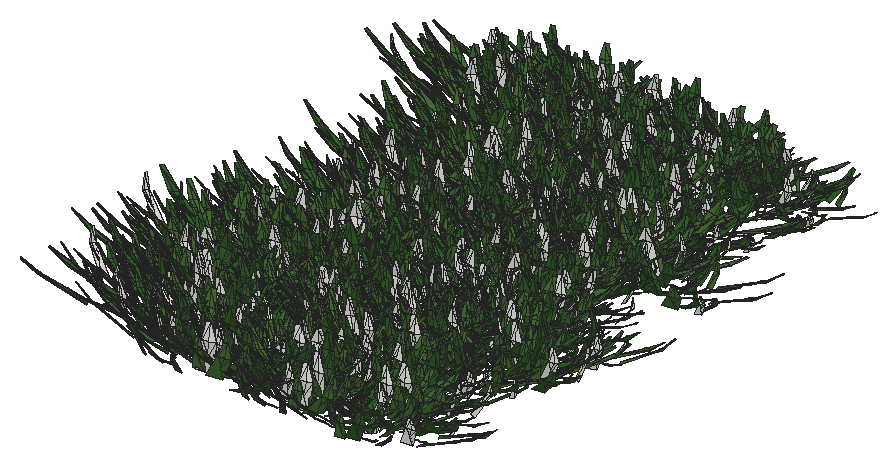
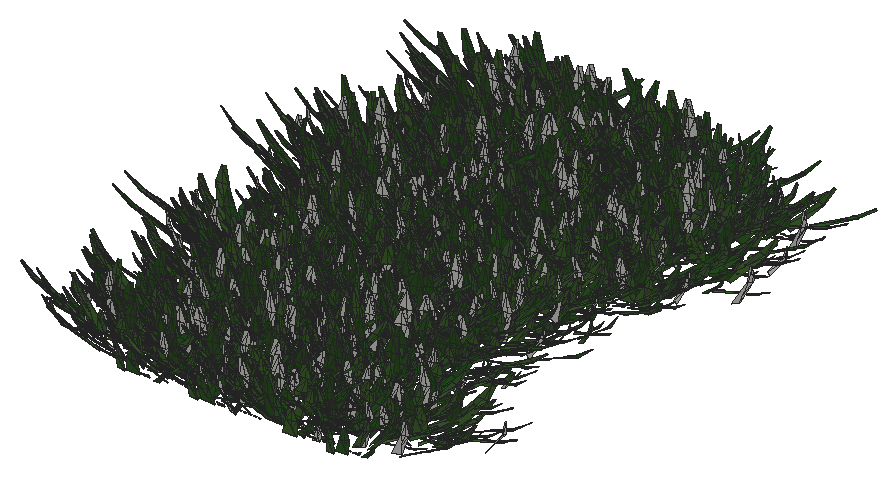
# SketchUp Ruby script. Lengths in inches.
U = 1.inch
M = Sketchup.active_model
def pt(a) = Geom::Point3d.new(a.map { |v| v * U })
def face(e, loops, mat)
  f = e.add_face(loops[0].map { |a| pt(a) })
  loops[1..].each { |l| e.add_face(l.map { |a| pt(a) }).erase! }
  f.material = f.back_material = mat if mat
  f
end
# faces: each face lists its corners as indices into pts; further lists are holes
def faces(e, pts, list, mat = nil) = list.each { |f| face(e, (f[0].is_a?(Array) ? f : [f]).map { |l| l.map { |i| pts[i] } }, mat) }
# xy, xz, yz: faces in a plane at the given z, y or x. An outline is a flat list of corners, or four numbers for a rectangle; further outlines are holes
def ring(l) = l.size == 4 ? [[l[0], l[1]], [l[2], l[1]], [l[2], l[3]], [l[0], l[3]]] : l.each_slice(2).to_a
def flat(e, list, mat, &to3) = list.each { |f| face(e, (f[0].is_a?(Array) ? f : [f]).map { |l| ring(l).map { |u, v| to3.(u, v) } }, mat) }
def xy(e, z, list, mat = nil) = flat(e, list, mat) { |x, y| [x, y, z] }
def xz(e, y, list, mat = nil) = flat(e, list, mat) { |x, z| [x, y, z] }
def yz(e, x, list, mat = nil) = flat(e, list, mat) { |y, z| [x, y, z] }
def lines(e, pts, list) = list.each { |a, b| e.add_line(pt(pts[a]), pt(pts[b])) }
# prism: a flat outline (further loops are holes) pulled along v
def prism(e, loops, v, mat = nil)
  f = face(e, loops, mat); d = Geom::Vector3d.new(v.map { |x| x * U })
  f.pushpull(f.normal.samedirection?(d) ? d.length : -d.length)
end
def box(e, o, s, mat = nil) = prism(e, [[o, [o[0] + s[0], o[1], o[2]], [o[0] + s[0], o[1] + s[1], o[2]], [o[0], o[1] + s[1], o[2]]]], [0, 0, s[2]], mat)
def at(x, y, z, deg = 0) = Geom::Transformation.translation(pt([x, y, z])) * Geom::Transformation.rotation(ORIGIN, Z_AXIS, deg.degrees)
def axes(o, x, y, z) = Geom::Transformation.new([*x, 0, *y, 0, *z, 0, *pt(o).to_a, 1])
def part(name) = M.definitions.add(name)
# library, detail: a bought-in or finely detailed component or shape, given as its bounding box
def library(name, o, s) = part(name).tap { |d| box(d.entities, o, s) }
def detail(e, o, s) = box(e.add_group.entities, o, s)
def put(e, d, t, mat = nil) = e.add_instance(d, t).tap { |i| i.material = mat if mat }
def group(e, t, mat = nil) = e.add_group.tap { |g| g.transformation = t; g.material = mat if mat }.entities
root = M.entities
M.materials.add("Material82").color = [68, 110, 58]
M.materials.add("Material83").color = [48, 90, 38]
M.materials.add("Material84").color = [68, 110, 48]
M.materials.add("Material85").color = [48, 90, 48]
M.materials.add("Material86").color = [58, 110, 58]
M.materials.add("Material87").color = [58, 90, 38]
M.materials.add("Material88").color = [68, 100, 58]
M.materials.add("Material89").color = [48, 100, 38]
c1 = part("grass00")
p = [[-0.6875,0.15,0],[-0.56,0.08,5.52],[-0.04,0.03,2.76],[0.48,-0.02,0],[0.35,-0.02,5.52],[-0.1,-0.14,5.52],
  [-0.12,0.65,8.37],[-0.42,0.65,8.37]]
faces(c1.entities,p,[[0,1,2,3],[3,2,4],[1,5,2],[5,4,2],[1,6,5],[4,5,6],[7,6,1]])
c2 = part("Group16\#1")
put(c2.entities,c1,axes([1.44,-0.61,-0.01],[0.05352,0.12609,0],[-0.10704,0.04543,0.07239],[0.06664,-0.02828,0.11628]),"Material85")
put(c2.entities,c1,axes([0.76,-0.15,-0.01],[0.04676,0.24062,0],[-0.23162,0.04501,0.06642],[0.0652,-0.01267,0.23595]),"Material82")
put(c2.entities,c1,axes([0.79,0.01,-0.01],[-0.00606,0.34651,0],[-0.34381,-0.00602,0.0432],[0.04319,0.00076,0.34386]))
put(c2.entities,c1,axes([1,0.23,-0.01],[-0.07192,0.31144,0],[-0.28722,-0.06632,0.1236],[0.12043,0.02781,0.29478]),"Material84")
put(c2.entities,c1,axes([1.66,0.77,-0.01],[-0.13828,0.29651,0],[-0.21551,-0.1005,0.22471],[0.20365,0.09498,0.23779]),"Material89")
put(c2.entities,c1,axes([0.6875,0.52,-0.01],[-0.18126,0.24051,0],[-0.22746,-0.17142,0.09788],[0.07817,0.05891,0.28481]),"Material84")
put(c2.entities,c1,axes([0.68,0.78,-0.01],[-0.215,0.18688,0],[-0.12385,-0.14248,0.21334],[0.13995,0.16101,0.18878]),"Material82")
put(c2.entities,c1,axes([0.56,1,-0.01],[-0.13756,0.07624,0],[-0.06159,-0.11112,0.0927],[0.04494,0.08108,0.12705]),"Material84")
put(c2.entities,c1,axes([0.2,0.64,-0.01],[-0.23729,0.07254,0],[-0.05711,-0.18681,0.153],[0.04473,0.14632,0.19535]),"Material89")
put(c2.entities,c1,axes([0.0625,0.72,-0.01],[-0.28874,0.02525,0],[-0.02179,-0.24916,0.14647],[0.01276,0.14591,0.25012]),"Material82")
put(c2.entities,c1,axes([-0.08,0.62,-0.01],[-0.34089,-0.04187,0],[0.03255,-0.26504,0.216],[-0.02633,0.21439,0.26703]),"Material89")
put(c2.entities,c1,axes([-0.34,0.98,-0.01],[-0.14314,-0.0493,0],[0.04397,-0.12769,0.06843],[-0.02228,0.0647,0.13505]),"Material89")
put(c2.entities,c1,axes([-0.87,1.45,-0.01],[-0.23488,-0.14114,0],[0.13761,-0.22901,0.06087],[-0.03135,0.05217,0.26717]))
put(c2.entities,c1,axes([-0.72,0.77,-0.01],[-0.14208,-0.13251,0],[0.07209,-0.0773,0.16301],[-0.11118,0.11922,0.1057]),"Material89")
put(c2.entities,c1,axes([-0.62,0.43,-0.01],[-0.14845,-0.21203,0],[0.18654,-0.13061,0.12304],[-0.10079,0.07057,0.22772]),"Material82")
put(c2.entities,c1,axes([-0.68,0.29,-0.01],[-0.13639,-0.32136,0],[0.31723,-0.13464,0.05579],[-0.05136,0.0218,0.34462]),"Material83")
put(c2.entities,c1,axes([-0.64,0.125,-0.01],[-0.0458,-0.23569,0],[0.22124,-0.043,0.08276],[-0.08124,0.01579,0.22538]),"Material86")
put(c2.entities,c1,axes([-1.6,-0.03,-0.01],[0.00576,-0.32897,0],[0.27526,0.00482,0.18018],[-0.18015,-0.00315,0.2753]),"Material84")
put(c2.entities,c1,axes([-1.36,-0.31,-0.01],[0.05718,-0.24765,0],[0.18172,0.04196,0.17267],[-0.16825,-0.03885,0.1865]),"Material89")
put(c2.entities,c1,axes([-1.54,-0.72,-0.01],[0.06537,-0.14017,0],[0.13555,0.06321,0.03939],[-0.0357,-0.01665,0.14956]))
put(c2.entities,c1,axes([-1.19,-0.9,-0.01],[0.09597,-0.12735,0],[0.11214,0.08451,0.07557],[-0.06035,-0.04548,0.14042]),"Material88")
put(c2.entities,c1,axes([-0.47,-0.54,-0.01],[0.11588,-0.10072,0],[0.0618,0.0711,0.12124],[-0.07953,-0.0915,0.0942]))
put(c2.entities,c1,axes([-0.47,-0.84,-0.01],[0.11927,-0.0661,0],[0.06603,0.11913,0.00646],[-0.00313,-0.00565,0.13621]),"Material84")
put(c2.entities,c1,axes([-0.38,-1.24,-0.01],[0.28037,-0.08571,0],[0.0618,0.20215,0.20315],[-0.05939,-0.19428,0.21139]),"Material88")
put(c2.entities,c1,axes([-0.06,-0.66,-0.01],[0.22719,-0.01987,0],[0.01247,0.14255,0.17758],[-0.01547,-0.17691,0.1431]),"Material87")
put(c2.entities,c1,axes([0.11,-0.89,-0.01],[0.14882,0.01828,0],[-0.01058,0.08611,0.12229],[0.01491,-0.12138,0.08676]),"Material85")
put(c2.entities,c1,axes([0.25,-0.72,-0.01],[0.20481,0.07053,0],[-0.06206,0.18022,0.10291],[0.03351,-0.0973,0.1906]),"Material85")
put(c2.entities,c1,axes([0.85,-1.42,-0.01],[0.16481,0.09904,0],[-0.09472,0.15762,0.05616],[0.02893,-0.04814,0.18389]),"Material84")
put(c2.entities,c1,axes([1.01,-1.09,-0.01],[0.21858,0.20385,0],[-0.17495,0.1876,0.15339],[0.10462,-0.11218,0.25652]),"Material89")
put(c2.entities,c1,axes([1.01,-0.71,-0.01],[0.08733,0.12473,0],[-0.06445,0.04512,0.13037],[0.1068,-0.07477,0.07867]),"Material85")
c3 = part("Group15\#1")
put(c3.entities,c2,at(0,0,0))
c4 = part("3darcstudiotree_grass00\#1")
put(c4.entities,c3,at(0,0,0))
put(root,c4,axes([1732.73,956.72,-29.74],[2.78328,1.41625,0],[-3.60575,1.10211,-0.03267],[-0.14651,0.04478,1.93988]))
put(root,c4,axes([1732.9,991.06,-29.74],[1.42302,1.52353,0],[-4.19442,0.60932,-0.04046],[-0.17686,0.02569,1.56076]))
put(root,c4,axes([1733,952.4375,-29.74],[0.02685,1.39613,0],[-4.67009,0.01397,-0.03677],[-0.14547,0.00044,1.38481]))
put(root,c4,axes([1734.73,944.23,-29.74],[-3.90096,-0.14279,0],[0.42836,-1.82008,-0.06502],[0.0247,-0.10495,1.42798]))
put(root,c4,axes([1733.78,961.63,-29.74],[-0.58657,1.2788,0],[-3.43074,-0.24475,-0.01415],[-0.07642,-0.00545,1.43376]))
put(root,c4,axes([1734.81,950.95,-29.74],[1.37504,-1.64012,0],[4.21946,0.55019,-0.04027],[0.19656,0.02563,1.71232]))
put(root,c4,axes([1734.89,992.02,-29.74],[3.4755,-0.56156,0],[1.30477,1.25594,-0.00746],[0.01674,0.01612,1.52751]))
put(root,c4,axes([1734.32,945.99,-29.74],[2.831,1.13552,0],[-3.26481,1.26594,-0.00938],[-0.03813,0.01479,1.95578]))
put(root,c4,axes([1737,963.81,-29.74],[-0.94888,-1.39552,0],[4.53946,-0.48005,-0.04199],[0.20499,-0.02168,1.7807]))
put(root,c4,axes([1737.37,970.1875,-29.74],[-2.56412,-1.04956,0],[2.92241,-1.11041,-0.03217],[0.12075,-0.04588,1.58546]))
put(root,c4,axes([1737.06,950.78,-29.74],[-4.23608,0.30685,0],[-0.85226,-1.82987,-0.05609],[-0.05564,-0.11947,1.94158]))
put(root,c4,axes([1737.32,960.52,-29.74],[-3.83901,-0.76558,0],[1.48905,-1.16132,-0.0255],[0.09039,-0.0705,1.94297]))
put(root,c4,axes([1737,996.64,-29.74],[-3.22115,0.33319,0],[-1.15137,-1.73117,-0.03948],[-0.04657,-0.07003,1.58152]))
put(root,c4,axes([1736.98,988.74,-29.74],[-3.56945,0.98002,0],[-2.54129,-1.43957,-0.02528],[-0.0766,-0.04339,1.76765]))
put(root,c4,axes([1736.73,947.1,-29.74],[0.13943,1.51336,0],[-3.52829,0.05056,-0.04285],[-0.2957,0.00424,1.82733]))
put(root,c4,axes([1736.92,986.46,-29.74],[3.38923,-0.39007,0],[1.26949,1.71555,-0.04654],[0.05157,0.06969,1.34343]))
put(root,c4,axes([1736.65,994.52,-29.74],[3.63174,0.64343,0],[-1.49454,1.312,-0.04301],[-0.1083,0.09507,1.6797]))
put(root,c4,axes([1737.22,961.37,-29.74],[3.52935,-0.50726,0],[1.49485,1.61761,-0.06136],[0.11602,0.12555,1.80687]))
put(root,c4,axes([1738.61,948.92,-29.74],[-0.52019,-1.47295,0],[3.61124,-0.19836,-0.01078],[0.07028,-0.00386,1.79898]))
put(root,c4,axes([1738.97,972.49,-29.74],[-1.338,-1.30891,0],[3.60545,-0.57321,-0.00075],[0.00363,-0.00058,1.52674]))
put(root,c4,axes([1737.54,953.74,-29.74],[3.75686,0.07381,0],[-0.21994,1.74119,-0.00527],[-0.00126,0.00998,1.59512]))
put(root,c4,axes([1739.66,992.26,-29.74],[-1.97999,-1.67359,0],[3.87039,-0.71217,-0.01753],[0.07436,-0.01368,1.49864]))
put(root,c4,axes([1738.46,980.1,-29.74],[3.4977,-1.17788,0],[2.34178,1.08154,-0.01134],[0.04108,0.01897,1.5074]))
put(root,c4,axes([1739.2,945.17,-29.74],[-4.29885,0.51765,0],[-1.3445,-1.73657,-0.03433],[-0.03931,-0.05078,1.35329]))
put(root,c4,axes([1738.99,974.28,-29.74],[-3.01219,1.1686,0],[-2.47695,-0.99299,-0.0233],[-0.1132,-0.04538,1.83382]))
put(root,c4,axes([1738.73,977.27,-29.74],[-0.71352,1.56405,0],[-4.14814,-0.29432,-0.02584],[-0.10481,-0.00744,1.30174]))
put(root,c4,axes([1739.89,983.25,-29.74],[1.98892,-1.13086,0],[3.89758,1.06614,-0.02169],[0.07891,0.02158,1.57389]))
put(root,c4,axes([1739.04,955.29,-29.74],[-0.64515,1.28427,0],[-4.09885,-0.32024,-0.03573],[-0.18751,-0.01465,1.67549]))
put(root,c4,axes([1740.4375,941.89,-29.74],[-3.41936,-0.32293,0],[0.80872,-1.33182,-0.00326],[0.00565,-0.00931,1.93944]))
put(root,c4,axes([1738.94,957.94,-29.74],[2.80686,0.98493,0],[-2.35719,1.04478,-0.00943],[-0.03285,0.01456,1.39243]))
put(root,c4,axes([1739.68,965.74,-29.74],[-0.90085,1.67926,0],[-4.44806,-0.37112,-0.05558],[-0.25392,-0.02119,1.59125]))
put(root,c4,axes([1740.39,989.9,-29.74],[1.68218,-1.47179,0],[3.03421,0.53937,-0.02223],[0.13236,0.02353,1.62899]))
put(root,c4,axes([1740.48,980.9,-29.74],[3.50844,-0.55754,0],[1.25662,1.22985,-0.02314],[0.04614,0.04516,1.34449]))
put(root,c4,axes([1739.95,968.23,-29.74],[1.7612,1.59038,0],[-3.40002,0.5856,-0.01938],[-0.1015,0.01748,1.58937]))
put(root,c4,axes([1742.14,960.2,-29.74],[-1.60359,-1.29455,0],[3.30864,-0.63743,-0.0349],[0.20941,-0.04034,1.84302]))
put(root,c4,axes([1742.72,973.52,-29.74],[-3.86108,-0.00922,0],[0.0279,-1.817,-0.0591],[0.00158,-0.1028,1.52309]))
put(root,c4,axes([1742.93,969.26,-29.74],[-4.30049,-0.14117,0],[0.33609,-1.59238,-0.036],[0.01919,-0.09092,1.9513]))
put(root,c4,axes([1742.7,985.21,-29.74],[1.67099,-1.73753,0],[3.10475,0.46439,-0.00605],[0.0444,0.00664,1.95327]))
put(root,c4,axes([1742.79,997.1,-29.74],[1.32812,-1.21732,0],[3.65511,0.62022,-0.02985],[0.14197,0.02409,1.54439]))
put(root,c4,axes([1742.5,980.74,-29.74],[0.83797,-1.39271,0],[3.20742,0.30015,-0.04624],[0.35526,0.03324,1.95114]))
put(root,c4,axes([1742.49,990.49,-29.74],[-2.03219,1.40442,0],[-2.95743,-0.66557,-0.04437],[-0.22116,-0.04977,1.46464]))
put(root,c4,axes([1742.14,948.75,-29.74],[-0.97814,1.51943,0],[-3.80237,-0.3807,-0.01715],[-0.08253,-0.00826,1.46021]))
put(root,c4,axes([1743.71,974.73,-29.74],[-0.67683,-1.69031,0],[4.16932,-0.25965,-0.01303],[0.08012,-0.00499,1.96953]))
put(root,c4,axes([1743.39,940.56,-29.74],[1.22394,-1.54587,0],[4.34445,0.53497,-0.04262],[0.21661,0.02667,1.81655]))
put(root,c4,axes([1743.99,963.42,-29.74],[-4.29208,0.36507,0],[-0.8528,-1.5594,-0.00845],[-0.00798,-0.0146,1.35873]))
put(root,c4,axes([1743.45,953.15,-29.74],[-2.45653,1.59128,0],[-3.13753,-0.75331,-0.03488],[-0.14833,-0.03561,1.37068]))
put(root,c4,axes([1743,958.01,-29.74],[3.38301,-0.17676,0],[0.47183,1.40447,-0.04905],[0.03546,0.10554,1.48186]))
put(root,c4,axes([1743.66,966.33,-29.74],[-2.91157,1.30067,0],[-2.86972,-0.9991,-0.01581],[-0.05499,-0.01914,1.33135]))
put(root,c4,axes([1743.625,945.11,-29.74],[3.20776,-0.47754,0],[1.28857,1.34619,-0.04981],[0.10847,0.11332,1.68613]))
put(root,c4,axes([1744.86,945.81,-29.74],[-0.83396,-1.47678,0],[3.24144,-0.28469,-0.00779],[0.04244,-0.00373,1.38852]))
put(root,c4,axes([1744.88,971.18,-29.74],[-2.06199,-1.44492,0],[3.43124,-0.76156,-0.05229],[0.2544,-0.05646,1.64764]))
put(root,c4,axes([1744.98,955.42,-29.74],[0.41064,-1.32496,0],[4.30887,0.2077,-0.02785],[0.12721,0.00613,1.49696]))
put(root,c4,axes([1744.07,962.01,-29.74],[-2.19345,1.65823,0],[-4.03021,-0.82913,-0.04188],[-0.20563,-0.0423,1.88687]))
put(root,c4,axes([1743.46,983.93,-29.74],[2.88531,0.9286,0],[-2.55752,1.23593,-0.03119],[-0.12387,0.05986,1.90467]))
put(root,c4,axes([1744.59,994.86,-29.74],[-1.83042,1.58988,0],[-3.0568,-0.54735,-0.0444],[-0.26156,-0.04683,1.62807]))
put(root,c4,axes([1744.93,976.625,-29.74],[-2.26778,1.36387,0],[-3.7802,-0.97758,-0.05216],[-0.16857,-0.04359,1.30947]))
put(root,c4,axes([1744.93,978.76,-29.74],[-1.84352,1.61201,0],[-4.26993,-0.75947,-0.03185],[-0.15055,-0.02678,1.82087]))
put(root,c4,axes([1745.02,951.04,-29.74],[2.07706,1.01263,0],[-2.63538,0.84072,-0.02717],[-0.1514,0.0483,1.82093]))
put(root,c4,axes([1745.12,942.21,-29.74],[3.46015,0.38109,0],[-0.88814,1.25417,-0.03829],[-0.05842,0.0825,1.40372]))
put(root,c4,axes([1745.64,988.56,-29.74],[3.97524,-0.29729,0],[0.87691,1.8237,-0.05959],[0.04913,0.10217,1.56123]))
put(root,c4,axes([1745.76,991.9375,-29.74],[0.81482,1.77329,0],[-4.44159,0.31742,-0.02342],[-0.11628,0.00831,1.70718]))
put(root,c4,axes([1747.86,941.86,-29.74],[-3.61082,-0.39433,0],[1.20081,-1.71014,-0.02644],[0.03989,-0.05681,1.9068]))
put(root,c4,axes([1748.57,981.76,-29.74],[-3.88555,-0.79581,0],[2.02489,-1.53765,-0.03725],[0.08107,-0.06156,1.55507]))
put(root,c4,axes([1747.78,994.47,-29.74],[-2.70631,1.45447,0],[-3.636,-1.05223,-0.06171],[-0.25363,-0.0734,1.72322]))
put(root,c4,axes([1747.52,987.51,-29.74],[1.70731,1.1244,0],[-2.88773,0.68196,-0.04808],[-0.30467,0.07195,1.86326]))
put(root,c4,axes([1747.49,970.15,-29.74],[4.38861,-0.21228,0],[0.43057,1.38444,-0.03723],[0.02239,0.072,1.30959]))
put(root,c4,axes([1748.84,990.03,-29.74],[0.3333,-1.68825,0],[3.84573,0.11808,-0.01871],[0.11577,0.00355,1.79426]))
put(root,c4,axes([1749.36,973.2,-29.74],[-2.17802,-1.23467,0],[3.55396,-0.97507,-0.03629],[0.13271,-0.03641,1.44541]))
put(root,c4,axes([1749.45,968.3,-29.74],[-2.33047,-0.97071,0],[3.43186,-1.28143,-0.06171],[0.20646,-0.07709,1.63202]))
put(root,c4,axes([1749.65,946.09,-29.74],[0.8669,-1.63737,0],[4.38165,0.36081,-0.01659],[0.07514,0.00619,1.55232]))
put(root,c4,axes([1750.2,984.53,-29.74],[-4.08688,-0.61044,0],[1.62889,-1.6961,-0.00084],[0.00115,-0.0012,1.34285]))
put(root,c4,axes([1749.41,979.54,-29.74],[-2.729,0.78907,0],[-2.0311,-1.09252,-0.03589],[-0.15909,-0.08558,1.93035]))
put(root,c4,axes([1748.87,977.77,-29.74],[3.45505,-0.2676,0],[0.73895,1.48387,-0.00241],[0.00289,0.0058,1.79003]))
put(root,c4,axes([1749.36,975.52,-29.74],[-1.50877,1.48911,0],[-3.61563,-0.56976,-0.0529],[-0.26655,-0.042,1.58349]))
put(root,c4,axes([1748.85,956.99,-29.74],[1.39252,1.41751,0],[-3.18673,0.48689,-0.02409],[-0.14094,0.02153,1.60735]))
put(root,c4,axes([1748.74,944.65,-29.74],[4.57837,0.42186,0],[-0.79113,1.33536,-0.04207],[-0.04884,0.08244,1.32997]))
put(root,c4,axes([1749.98,952.64,-29.74],[-2.78854,1.36928,0],[-2.88748,-0.91457,-0.04358],[-0.20411,-0.06465,1.66757]))
put(root,c4,axes([1749.28,966.02,-29.74],[3.59081,0.56064,0],[-1.39714,1.39174,-0.03237],[-0.06842,0.06816,1.63378]))
put(root,c4,axes([1750.4,996.53,-29.74],[-3.54904,1.16368,0],[-2.54993,-1.20953,-0.00935],[-0.03236,-0.01535,1.61847]))
put(root,c4,axes([1750.21,963.43,-29.74],[3.39127,-1.14999,0],[2.14538,0.98397,-0.0226],[0.09906,0.04544,1.65792]))
put(root,c4,axes([1751.34,986.53,-29.74],[-4.21718,-0.04667,0],[0.09647,-1.35575,-0.03959],[0.00846,-0.11883,1.96257]))
put(root,c4,axes([1749.8125,962,-29.74],[4.10063,0.83805,0],[-2.12312,1.61572,-0.0509],[-0.10915,0.08307,1.61215]))
put(root,c4,axes([1750.5,960.24,-29.74],[3.6923,-0.26906,0],[0.83055,1.77269,-0.01263],[0.0116,0.02476,1.73191]))
put(root,c4,axes([1751.18,951.2,-29.74],[2.76982,-1.52047,0],[2.85461,0.80878,-0.0087],[0.04308,0.01221,1.60603]))
put(root,c4,axes([1751.42,955.36,-29.74],[3.07151,-0.57195,0],[1.60637,1.34169,-0.03456],[0.08725,0.07287,1.66747]))
put(root,c4,axes([1751.51,991.79,-29.74],[-0.75802,1.26839,0],[-3.28645,-0.30547,-0.04738],[-0.26314,-0.02446,1.4441]))
put(root,c4,axes([1750.82,949.48,-29.74],[2.67266,1.37649,0],[-3.28703,0.99263,-0.02004],[-0.06999,0.02114,1.3651]))
put(root,c4,axes([1753.08,996.91,-29.74],[-3.58911,0.17625,0],[-0.41421,-1.31187,-0.03309],[-0.02615,-0.08283,1.60704]))
put(root,c4,axes([1753.51,977.36,-29.74],[-3.53984,-0.54558,0],[1.35048,-1.36277,-0.02269],[0.0488,-0.04924,1.64292]))
put(root,c4,axes([1753.3,950.69,-29.74],[-4.11453,0.51388,0],[-1.13165,-1.40923,-0.01419],[-0.02668,-0.03323,1.75006]))
put(root,c4,axes([1753.125,940.28,-29.74],[2.17079,-1.3067,0],[3.53732,0.91396,-0.04807],[0.21538,0.05565,1.69791]))
put(root,c4,axes([1753.29,964.18,-29.74],[2.51974,-1.17528,0],[3.05999,1.02034,-0.03628],[0.13748,0.04584,1.49031]))
put(root,c4,axes([1754.1,985.46,-29.74],[-1.7024,-1.44396,0],[3.0538,-0.55996,-0.04244],[0.29035,-0.05324,1.90455]))
put(root,c4,axes([1754.11,942.14,-29.74],[1.63405,-1.64828,0],[3.24927,0.50099,-0.00888],[0.05923,0.00913,1.87213]))
put(root,c4,axes([1753.18,943.67,-29.74],[-1.01765,1.47435,0],[-4.56253,-0.4898,-0.0223],[-0.09653,-0.01036,1.58974]))
put(root,c4,axes([1754.8,992.84,-29.74],[-0.95803,-1.53129,0],[3.44538,-0.33525,-0.01268],[0.07432,-0.00723,1.60602]))
put(root,c4,axes([1755.26,965.75,-29.74],[-1.89774,-1.54823,0],[3.70179,-0.70571,-0.04214],[0.19197,-0.0366,1.55921]))
put(root,c4,axes([1754.53,987.47,-29.74],[-2.99752,0.92431,0],[-2.30263,-1.1614,-0.02144],[-0.09164,-0.04622,1.94421]))
put(root,c4,axes([1753.95,972.62,-29.74],[-0.63419,1.43243,0],[-3.71512,-0.25582,-0.03794],[-0.18856,-0.01298,1.42617]))
put(root,c4,axes([1754.52,948.26,-29.74],[-1.88196,1.3957,0],[-3.10758,-0.65171,-0.04799],[-0.32006,-0.06712,1.99284]))
put(root,c4,axes([1755.56,958.05,-29.74],[-1.98727,-1.58329,0],[3.14557,-0.61406,-0.01272],[0.05955,-0.01163,1.37453]))
put(root,c4,axes([1755.32,994.26,-29.74],[0.20206,-1.72347,0],[4.27325,0.07792,-0.04434],[0.21389,0.0039,1.54852]))
put(root,c4,axes([1756.19,959.95,-29.74],[-2.8282,-0.92386,0],[2.41261,-1.14869,-0.01497],[0.06145,-0.02926,1.82381]))
put(root,c4,axes([1754.75,945.9,-29.74],[-1.66334,1.46333,0],[-4.128,-0.72978,-0.00369],[-0.01567,-0.00277,1.57624]))
put(root,c4,axes([1755.49,955.7,-29.74],[-3.33624,1.28886,0],[-2.34327,-0.94338,-0.00183],[-0.00717,-0.00289,1.40539]))
put(root,c4,axes([1755.31,979.55,-29.74],[-2.28466,1.61729,0],[-3.8326,-0.84205,-0.0557],[-0.22938,-0.0504,1.55009]))
put(root,c4,axes([1756.59,983.32,-29.74],[-3.20918,-1.37059,0],[3.45166,-1.25697,-0.04946],[0.15315,-0.05577,1.48426]))
put(root,c4,axes([1756.4,969.96,-29.74],[-4.01536,-0.24387,0],[0.54359,-1.39202,-0.03709],[0.03558,-0.0911,1.68681]))
put(root,c4,axes([1756.06,968.24,-29.74],[-3.12054,0.56833,0],[-1.82234,-1.55622,-0.05064],[-0.09583,-0.08183,1.47033]))
put(root,c4,axes([1756.8,953.34,-29.74],[0.84647,-1.73268,0],[3.98325,0.30265,-0.00212],[0.01137,0.00086,1.6588]))
put(root,c4,axes([1756.21,990.19,-29.74],[3.17331,-0.50017,0],[1.66687,1.64477,-0.02256],[0.03879,0.03827,1.55958]))
put(root,c4,axes([1756.71,980.79,-29.74],[1.96831,-1.06776,0],[3.09361,0.88694,-0.02782],[0.14847,0.04257,1.89124]))
put(root,c4,axes([1756.17,962.45,-29.74],[2.38559,0.94842,0],[-2.99836,1.17298,-0.03885],[-0.13848,0.05417,1.58937]))
put(root,c4,axes([1756.72,975.67,-29.74],[3.11027,0.45791,0],[-1.48719,1.57105,-0.03179],[-0.06172,0.0652,1.76952]))
put(root,c4,axes([1758.63,970.99,-29.74],[-1.60231,-1.37282,0],[3.29691,-0.59848,-0.04546],[0.27162,-0.04931,1.78943]))
put(root,c4,axes([1758.99,973.1,-29.74],[0.96155,-1.39333,0],[3.31195,0.35548,-0.01758],[0.11319,0.01215,1.71636]))
put(root,c4,axes([1759.36,951.07,-29.74],[-3.63945,-0.58666,0],[1.30533,-1.25945,-0.04864],[0.1019,-0.09832,1.4319]))
put(root,c4,axes([1759.48,980.76,-29.74],[-1.71956,-1.37213,0],[4.12265,-0.80354,-0.04891],[0.23955,-0.04669,1.88309]))
put(root,c4,axes([1759.72,994.17,-29.74],[-3.8816,-0.56323,0],[1.5517,-1.6632,-0.01333],[0.02356,-0.02525,1.7245]))
put(root,c4,axes([1759.05,996.82,-29.74],[-3.46015,1.06405,0],[-2.06953,-1.04669,-0.02241],[-0.08068,-0.04081,1.47722]))
put(root,c4,axes([1759.3,948.7,-29.74],[-0.53843,-1.61653,0],[3.48383,-0.18047,-0.04534],[0.27707,-0.01435,1.62314]))
put(root,c4,axes([1759.68,961.84,-29.74],[0.02414,-1.32822,0],[3.48081,0.00984,-0.01704],[0.11733,0.00033,1.79616]))
put(root,c4,axes([1758.5,991.89,-29.74],[-1.06746,1.42925,0],[-3.87706,-0.45036,-0.01201],[-0.05554,-0.00645,1.46096]))
put(root,c4,axes([1760.08,967.68,-29.74],[-1.25473,-1.49042,0],[3.70912,-0.48565,-0.03393],[0.14523,-0.01902,1.3212]))
put(root,c4,axes([1758.98,940.29,-29.74],[4.07054,-0.47424,0],[1.26442,1.68794,-0.05518],[0.08285,0.1106,1.77288]))
put(root,c4,axes([1760.56,944.52,-29.74],[0.9992,-1.70874,0],[3.78612,0.34433,-0.00305],[0.01806,0.00164,1.76865]))
put(root,c4,axes([1759.75,964.62,-29.74],[-2.38248,1.06709,0],[-3.21771,-1.11734,-0.02335],[-0.09118,-0.03166,1.67208]))
put(root,c4,axes([1759.07,983.89,-29.74],[0.13535,1.36053,0],[-4.14262,0.0641,-0.00595],[-0.03791,0.00059,1.98232]))
put(root,c4,axes([1760.18,985.67,-29.74],[-3.44248,1.19972,0],[-2.84327,-1.26888,-0.04086],[-0.12277,-0.05479,1.46035]))
put(root,c4,axes([1760.42,965.7,-29.74],[2.50615,-1.32245,0],[2.94011,0.86656,-0.03861],[0.1979,0.05833,1.76068]))
put(root,c4,axes([1761.18,945.85,-29.74],[0.83554,-1.66698,0],[4.46376,0.34798,-0.04547],[0.22573,0.0176,1.72572]))
put(root,c4,axes([1760.97,990.65,-29.74],[-3.77371,1.09403,0],[-2.05317,-1.10148,-0.00523],[-0.01755,-0.00942,1.47184]))
put(root,c4,axes([1761,975.46,-29.74],[-3.53362,0.69285,0],[-1.78137,-1.413,-0.01143],[-0.02296,-0.01821,1.35283]))
put(root,c4,axes([1760.12,955.1,-29.74],[3.52761,0.55067,0],[-1.26989,1.26523,-0.04887],[-0.1287,0.12823,1.85053]))
put(root,c4,axes([1762,957.66,-29.74],[-4.29343,-0.7683,0],[1.85419,-1.61153,-0.00153],[0.00342,-0.00297,1.82565]))
put(root,c4,axes([1761.73,942.29,-29.74],[-4.08016,-0.15242,0],[0.34321,-1.42893,-0.02721],[0.0124,-0.05162,1.31849]))
put(root,c4,axes([1760.68,978.6,-29.74],[1.28441,1.48375,0],[-3.48852,0.46968,-0.04031],[-0.24472,0.03295,1.77227]))
put(root,c4,axes([1761.7,988.62,-29.74],[-3.58514,0.47051,0],[-1.41535,-1.67729,-0.02244],[-0.03437,-0.04073,1.62972]))
put(root,c4,axes([1762.03,960.4375,-29.74],[0.26653,-1.73376,0],[4.03869,0.09656,-0.02606],[0.1443,0.00345,1.68211]))
put(root,c4,axes([1761.76,953.66,-29.74],[-2.42435,1.35441,0],[-3.23148,-0.89962,-0.04566],[-0.20763,-0.0578,1.65042]))
put(root,c4,axes([1762.52,977.57,-29.74],[3.81611,-0.29546,0],[0.81359,1.63432,-0.02697],[0.02626,0.05275,1.59996]))
put(root,c4,axes([1764.79,962.01,-29.74],[-4.03021,-0.53258,0],[1.1352,-1.33605,-0.02118],[0.04192,-0.04934,1.66873]))
put(root,c4,axes([1765.26,956.72,-29.74],[0.48715,-1.38403,0],[3.63737,0.19912,-0.0013],[0.00869,0.00048,1.85519]))
put(root,c4,axes([1764.63,993.95,-29.74],[-1.21919,1.74404,0],[-3.47137,-0.37742,-0.03305],[-0.15949,-0.01734,1.35106]))
put(root,c4,axes([1765.2,975.37,-29.74],[-2.03127,1.47153,0],[-3.87167,-0.83121,-0.05406],[-0.22119,-0.04749,1.53936]))
